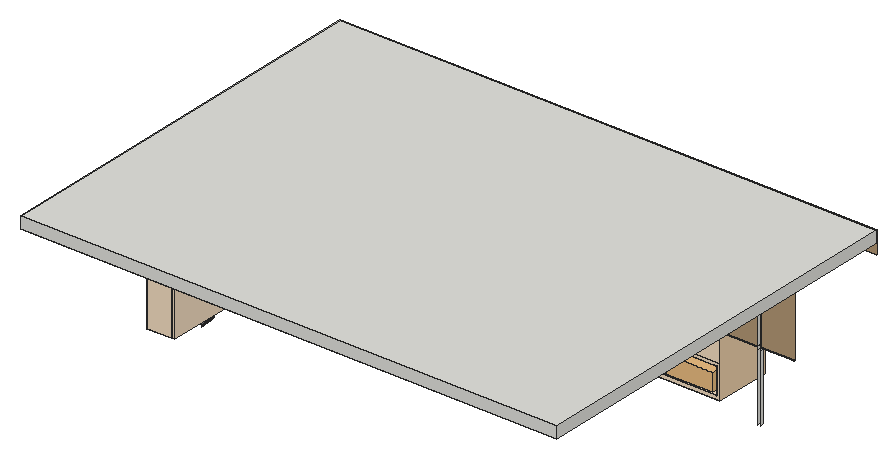
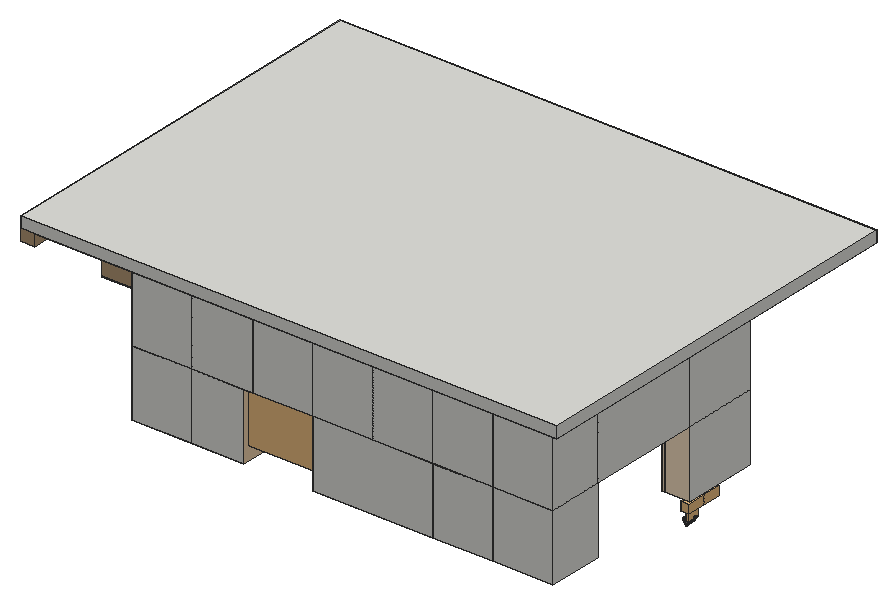
# SketchUp Ruby script. Lengths in inches.
U = 1.inch
M = Sketchup.active_model
def pt(a) = Geom::Point3d.new(a.map { |v| v * U })
def face(e, loops, mat)
  f = e.add_face(loops[0].map { |a| pt(a) })
  loops[1..].each { |l| e.add_face(l.map { |a| pt(a) }).erase! }
  f.material = f.back_material = mat if mat
  f
end
# faces: each face lists its corners as indices into pts; further lists are holes
def faces(e, pts, list, mat = nil) = list.each { |f| face(e, (f[0].is_a?(Array) ? f : [f]).map { |l| l.map { |i| pts[i] } }, mat) }
# xy, xz, yz: faces in a plane at the given z, y or x. An outline is a flat list of corners, or four numbers for a rectangle; further outlines are holes
def ring(l) = l.size == 4 ? [[l[0], l[1]], [l[2], l[1]], [l[2], l[3]], [l[0], l[3]]] : l.each_slice(2).to_a
def flat(e, list, mat, &to3) = list.each { |f| face(e, (f[0].is_a?(Array) ? f : [f]).map { |l| ring(l).map { |u, v| to3.(u, v) } }, mat) }
def xy(e, z, list, mat = nil) = flat(e, list, mat) { |x, y| [x, y, z] }
def xz(e, y, list, mat = nil) = flat(e, list, mat) { |x, z| [x, y, z] }
def yz(e, x, list, mat = nil) = flat(e, list, mat) { |y, z| [x, y, z] }
def lines(e, pts, list) = list.each { |a, b| e.add_line(pt(pts[a]), pt(pts[b])) }
# prism: a flat outline (further loops are holes) pulled along v
def prism(e, loops, v, mat = nil)
  f = face(e, loops, mat); d = Geom::Vector3d.new(v.map { |x| x * U })
  f.pushpull(f.normal.samedirection?(d) ? d.length : -d.length)
end
def box(e, o, s, mat = nil) = prism(e, [[o, [o[0] + s[0], o[1], o[2]], [o[0] + s[0], o[1] + s[1], o[2]], [o[0], o[1] + s[1], o[2]]]], [0, 0, s[2]], mat)
def at(x, y, z, deg = 0) = Geom::Transformation.translation(pt([x, y, z])) * Geom::Transformation.rotation(ORIGIN, Z_AXIS, deg.degrees)
def axes(o, x, y, z) = Geom::Transformation.new([*x, 0, *y, 0, *z, 0, *pt(o).to_a, 1])
def part(name) = M.definitions.add(name)
# library, detail: a bought-in or finely detailed component or shape, given as its bounding box
def library(name, o, s) = part(name).tap { |d| box(d.entities, o, s) }
def detail(e, o, s) = box(e.add_group.entities, o, s)
def put(e, d, t, mat = nil) = e.add_instance(d, t).tap { |i| i.material = mat if mat }
def group(e, t, mat = nil) = e.add_group.tap { |g| g.transformation = t; g.material = mat if mat }.entities
root = M.entities
M.materials.add("Generic").color = [180, 152, 118]
M.materials.add("Generic\#1").color = [237, 208, 170]
M.materials.add("Generic\#2").color = [244, 221, 193]
M.materials.add("[Color M00]").color = [255, 255, 255]
M.materials.add("agda_07_riverina_milk").color = [107, 143, 172]
M.materials.add("go trang").color = [128, 128, 128]
c1 = library("Hanging towel rail",[-9.5,0,-6.64],[9.89,2.15,7.51])
c2 = library("Towel rack",[0,0,0],[10.04,4.25,4.73])
c3 = library("place setting",[6.69,0,0],[21.5,21.5,5.53])
c4 = library("AutoSave_platos+BOWLS",[0,0,0],[6.24,6.24,7.68])
c5 = library("Group\#200",[0,0,0],[25.42,9.79,9.57])
c6 = library("Group\#201",[0,0,0],[3.49,3.49,6.7])
c7 = library("Group\#202",[0,0,0],[3.49,3.49,6.7])
c8 = library("Group\#203",[0,0,0],[3.49,3.49,6.7])
c9 = library("chimney",[0,0,0],[35.95,27.65,32.08])
c10 = library("Group\#513",[0,0,0],[2.91,2.91,4.14])
c11 = part("Component\#71")
xz(c11.entities,0,[[0,0,14.99,43.42]],"agda_07_riverina_milk")
xz(c11.entities,7.5,[[0,46.48,14.99,46.48,14.99,48.87,13.76,50.13,1.23,50.13,0,48.87]],"agda_07_riverina_milk")
xz(c11.entities,14.99,[[0,0,14.99,43.42]],"agda_07_riverina_milk")
yz(c11.entities,0,[[0,0,14.99,43.42]],"agda_07_riverina_milk")
yz(c11.entities,14.99,[[0,0,14.99,43.42]],"agda_07_riverina_milk")
p = [[1.53,7.5,46.07],[0,14.99,43.42],[0,0,43.42],[14.99,0,43.42],[14.99,7.5,46.48],[0,7.5,46.48],
  [13.46,7.5,46.07],[14.99,14.99,43.42]]
faces(c11.entities,p,[[0,1,2],[3,4,5,2],[5,0,2],[6,3,7],[6,4,3],[1,5,4,7],[0,5,1],[4,6,7]],"agda_07_riverina_milk")
c12 = part("Component\#69")
xy(c12.entities,0,[[7.08,5.17,4.88,7.37,4.88,9.5625,12.88,9.5625,12.88,7.37,10.68,5.17]],"agda_07_riverina_milk")
xy(c12.entities,29.07,[[4.98,0.48,12.43,0.48,16.97,5.02,16.97,9.5625,0.44,9.5625,0.44,5.02]],"agda_07_riverina_milk")
xy(c12.entities,30.1,[[4.78,0,12.63,0,17.41,4.78,17.41,9.5625,16.97,9.5625,16.97,5.02,12.43,0.48,4.98,0.48,0.44,5.02,0.44,9.5625,0,9.5625,0,4.78]],"agda_07_riverina_milk")
xz(c12.entities,0.48,[[4.98,29.07,12.43,30.1]],"agda_07_riverina_milk")
yz(c12.entities,0.44,[[5.02,29.07,9.5625,30.1]],"agda_07_riverina_milk")
yz(c12.entities,16.97,[[5.02,29.07,9.5625,30.1]],"agda_07_riverina_milk")
p = [[6.09,2.51,5.81],[2.57,6.04,5.81],[4.88,7.37,0],[7.08,5.17,0],[10.68,5.17,0],[11.88,2.51,5.81],
  [12.88,7.37,0],[15.41,6.04,5.81],[2.57,9.5625,5.81],[4.88,9.5625,0],[12.88,9.5625,0],[15.41,9.5625,5.81],
  [4.78,0,30.1],[0,4.78,30.1],[12.63,0,30.1],[17.41,4.78,30.1],[0,9.5625,30.1],[17.41,9.5625,30.1],
  [0.44,5.02,30.1],[4.98,0.48,30.1],[4.98,0.48,29.07],[0.44,5.02,29.07],[12.43,0.48,30.1],[16.97,5.02,30.1],
  [16.97,5.02,29.07],[12.43,0.48,29.07]]
faces(c12.entities,p,[[0,1,2,3],[4,5,0,3],[6,7,5,4],[1,8,9,2],[7,6,10,11],[0,12,13,1],[5,14,12,0],[7,15,14,5],
  [13,16,8,1],[15,7,11,17],[18,19,20,21],[22,23,24,25]],"agda_07_riverina_milk")
c13 = part("Groep\#9")
put(c13.entities,c12,axes([0,19.13,0],[1,0,0],[0,-1,0],[0,0,1]))
put(c13.entities,c12,at(0,0,0))
c14 = library("Group\#511",[0,0,-0.07],[6.38,6.25,7.32])
c15 = library("Tlon Light 450 Ceiling 152 006",[-8.86,-8.86,-3.78],[17.72,17.72,3.56])
xy(root,63.342,[[11.432,108.349,11.528,114.195]],"go trang")
xy(root,72,[[22.125,74.5,23.625,115]])
xy(root,72,[[73.875,177,139,207],[175.875,177,236.5,207]],"Generic\#1")
xy(root,72,[[9,74.5,22.125,115],[9,177,41.5,207],[41.5,177,73.875,207]],"Generic\#2")
xy(root,74.219,[[11.219,177,39.281,205.9375]],"Generic\#2")
xy(root,88.275,[[177.288,177,204,204.9375],[204,177,234.775,204.9375]],"Generic\#2")
xy(root,89,[[11.219,177,39.281,205.9375]],"Generic\#2")
xy(root,89.7,[[74.175,177,139,177.3]])
xy(root,90,[[73.875,177,74.175,177.3],[74.175,177,139,177.3]])
xy(root,90.5,[[11.219,177,39.281,205.9375]],"Generic\#2")
xy(root,105.781,[[38.6875,177,39.281,205.9375]])
xy(root,105.781,[[11.219,177,38.6875,205.9375]],"Generic\#2")
xy(root,108,[[23.625,74.5,23.625,115,9,115,9,177,38.6875,177,38.6875,74.5],[9,74.5,22.125,115],[22.125,74.5,23.625,115],[38.6875,74.5,41.1875,177],[9,177,41.5,207],
  [41.5,177,73.875,177.3],[74.175,177,139,177.3],[171.5,177,171.8,177.3],[171.8,177,175.875,177.3],[175.875,177,236.5,177.3],
  [41.5,177.3,73.875,207],[106.5,177.3,139,207],[171.5,177.3,175.875,207],[175.875,177.3,204,207],[204,177.3,236.5,207]])
xy(root,108,[[139.3,177,139.3,177.3,139,177.3,139,207,171.5,207,171.5,177]],"Generic\#1")
xy(root,108.3,[[41.5,177,73.875,177.3],[73.875,177,74,177.3],[74.3,177,106.5,177.3],[106.8,177,139,177.3],[171.8,177,204,177.3],
  [204.3,177,236.5,177.3]])
xy(root,109.724,[[239.5625,171,261.8125,171.3],[263.25,171,281.625,171.3]])
xy(root,110.024,[[239.5625,171,261.8125,171.3],[263.25,171,281.625,171.3]])
xy(root,144,[[9,74.5,38.6875,177],[38.6875,74.5,41.1875,177],[9,177,41.5,207],[41.5,177,74,207],[74.3,177,106.5,177,106.5,207,74,207,74,177.3,74.3,177.3],
  [106.8,177,139,177,139,207,106.5,207,106.5,177.3,106.8,177.3],[139.3,177,171.5,177,171.5,207,139,207,139,177.3,139.3,177.3],[171.8,177,204,177,204,207,171.5,207,171.5,177.3,171.8,177.3],[204.3,177,236.5,177,236.5,207,204,207,204,177.3,204.3,177.3]],"Generic\#2")
xy(root,150,[[9,9,9,207,239.5625,207,239.5625,182.261,33.739,182.261,33.739,24.739,264.948,24.739,261.8125,172.303,261.8125,172.375,263.25,172.375,263.25,171,281.625,171,281.625,207,289.6875,207,289.6875,9],[239.5625,171,239.5625,182.261,261.601,182.261,261.8125,172.303,261.8125,171],[263.25,171,263.25,172.375,261.8125,172.375,261.8125,172.303,261.601,182.261,239.5625,182.261,239.5625,207,281.625,207,281.625,171]])
xy(root,150,[[281.625,207,289.6875,216]],"Generic")
xy(root,150,[[0,0,0,216,281.625,216,281.625,207,9,207,9,9,289.6875,9,289.6875,0]],"[Color M00]")
xy(root,153.9375,[[33.739,24.739,33.739,182.261,239.5625,182.261,239.5625,171,261.8125,171,261.8125,172.303,264.948,24.739]])
xy(root,156,[[0,0,289.6875,216]])
xz(root,0,[[0,150,289.6875,156]])
xz(root,24.739,[[33.739,150,228.739,153.9375],[228.739,150,264.948,153.9375]])
xz(root,74.5,[[9,72,22.125,108],[22.125,72,23.625,108],[9,108,38.6875,144],[38.6875,108,41.1875,144]],"Generic\#2")
xz(root,108.349,[[[11.436,60.122,11.532,60.123,11.628,60.129,11.723,60.142,11.817,60.161,11.91,60.186,12.001,60.218,12.09,60.255,12.177,60.298,12.261,60.347,12.341,60.402,12.419,60.461,12.493,60.526,12.5625,60.595,12.628,60.669,12.689,60.747,12.745,60.829,12.796,60.915,12.601,60.516,12.716,60.735,12.822,60.96,12.918,61.189,12.948,61.285,12.972,61.383,12.989,61.483,13.001,61.583,13.007,61.684,13.007,61.785,13.001,61.886,12.989,61.987,12.971,62.086,12.947,62.184,12.917,62.28,12.882,62.374,12.841,62.466,12.794,62.554,12.743,62.64,12.686,62.721,12.625,62.799,12.559,62.873,12.489,62.942,12.415,63.006,12.338,63.066,12.257,63.12,12.173,63.169,12.086,63.211,11.997,63.249,11.906,63.28,11.8125,63.305,11.718,63.324,11.623,63.336,11.528,63.342,11.432,63.342,11.336,63.336,11.241,63.323,11.147,63.304,11.054,63.278,10.963,63.247,10.874,63.21,10.787,63.166,10.703,63.118,10.622,63.063,10.545,63.004,10.471,62.939,10.401,62.87,10.336,62.796,10.275,62.718,10.219,62.636,10.167,62.55,10.121,62.462,10.081,62.37,10.045,62.276,10.016,62.18,9.992,62.081,9.974,61.982,9.963,61.882,9.963,61.881,9.961,61.858,9.957,61.781,9.957,61.68,9.963,61.579,9.975,61.478,9.993,61.379,10.017,61.281,10.047,61.185,10.082,61.091,10.123,60.999,10.17,60.911,10.221,60.825,10.278,60.743,10.339,60.666,10.404,60.592,10.474,60.523,10.548,60.458,10.626,60.399,10.707,60.345,10.791,60.296,10.878,60.253,10.967,60.216,11.058,60.185,11.151,60.16,11.245,60.141,11.34,60.129],[11.482,61.122,11.446,61.124,11.409,61.127,11.374,61.133,11.338,61.142,11.303,61.152,11.269,61.165,11.236,61.18,11.203,61.198,11.172,61.217,11.142,61.239,11.114,61.262,11.086,61.288,11.061,61.315,11.037,61.344,11.014,61.374,10.994,61.406,10.975,61.439,10.959,61.473,10.945,61.508,10.932,61.544,10.922,61.581,10.914,61.618,10.909,61.656,10.905,61.694,10.904,61.732,10.905,61.771,10.909,61.809,10.914,61.847,10.922,61.884,10.932,61.921,10.945,61.957,10.959,61.992,10.975,62.026,10.994,62.059,11.014,62.091,11.037,62.121,11.061,62.15,11.086,62.177,11.114,62.202,11.142,62.226,11.172,62.247,11.203,62.267,11.236,62.284,11.269,62.3,11.303,62.3125,11.338,62.323,11.374,62.332,11.409,62.338,11.446,62.341,11.482,62.342,11.518,62.341,11.554,62.338,11.59,62.332,11.626,62.323,11.661,62.3125,11.695,62.3,11.728,62.284,11.76,62.267,11.792,62.247,11.822,62.226,11.85,62.202,11.878,62.177,11.903,62.15,11.927,62.121,11.95,62.091,11.97,62.059,11.988,62.026,12.005,61.992,12.019,61.957,12.032,61.921,12.042,61.884,12.05,61.847,12.055,61.809,12.059,61.771,12.06,61.732,12.059,61.694,12.055,61.656,12.05,61.618,12.042,61.581,12.032,61.544,12.019,61.508,12.005,61.473,11.988,61.439,11.97,61.406,11.95,61.374,11.927,61.344,11.903,61.315,11.878,61.288,11.85,61.262,11.822,61.239,11.792,61.217,11.76,61.198,11.728,61.18,11.695,61.165,11.661,61.152,11.626,61.142,11.59,61.133,11.554,61.127,11.518,61.124]],[12.601,60.516,12.716,60.735,12.822,60.96,12.918,61.189,12.883,61.095,12.843,61.003,12.796,60.915]],"go trang")
xz(root,114.195,[[[11.436,60.122,11.34,60.129,11.245,60.141,11.151,60.16,11.058,60.185,10.967,60.216,10.878,60.253,10.791,60.296,10.707,60.345,10.626,60.399,10.548,60.458,10.474,60.523,10.404,60.592,10.339,60.666,10.278,60.743,10.221,60.825,10.17,60.911,10.123,60.999,10.082,61.091,10.047,61.185,10.017,61.281,9.993,61.379,9.975,61.478,9.963,61.579,9.957,61.68,9.957,61.781,9.961,61.858,9.963,61.881,9.963,61.882,9.974,61.982,9.992,62.081,10.016,62.18,10.045,62.276,10.081,62.37,10.121,62.462,10.167,62.55,10.219,62.636,10.275,62.718,10.336,62.796,10.401,62.87,10.471,62.939,10.545,63.004,10.622,63.063,10.703,63.118,10.787,63.166,10.874,63.21,10.963,63.247,11.054,63.278,11.147,63.304,11.241,63.323,11.336,63.336,11.432,63.342,11.528,63.342,11.623,63.336,11.718,63.324,11.8125,63.305,11.906,63.28,11.997,63.249,12.086,63.211,12.173,63.169,12.257,63.12,12.338,63.066,12.415,63.006,12.489,62.942,12.559,62.873,12.625,62.799,12.686,62.721,12.743,62.64,12.794,62.554,12.841,62.466,12.882,62.374,12.917,62.28,12.947,62.184,12.971,62.086,12.989,61.987,13.001,61.886,13.007,61.785,13.007,61.684,13.001,61.583,12.989,61.483,12.972,61.383,12.948,61.285,12.918,61.189,12.883,61.095,12.843,61.003,12.796,60.915,12.745,60.829,12.689,60.747,12.628,60.669,12.5625,60.595,12.493,60.526,12.419,60.461,12.341,60.402,12.261,60.347,12.177,60.298,12.09,60.255,12.001,60.218,11.91,60.186,11.817,60.161,11.723,60.142,11.628,60.129,11.532,60.123],[11.482,61.122,11.518,61.124,11.554,61.127,11.59,61.133,11.626,61.142,11.661,61.152,11.695,61.165,11.728,61.18,11.76,61.198,11.792,61.217,11.822,61.239,11.85,61.262,11.878,61.288,11.903,61.315,11.927,61.344,11.95,61.374,11.97,61.406,11.988,61.439,12.005,61.473,12.019,61.508,12.032,61.544,12.042,61.581,12.05,61.618,12.055,61.656,12.059,61.694,12.06,61.732,12.059,61.771,12.055,61.809,12.05,61.847,12.042,61.884,12.032,61.921,12.019,61.957,12.005,61.992,11.988,62.026,11.97,62.059,11.95,62.091,11.927,62.121,11.903,62.15,11.878,62.177,11.85,62.202,11.822,62.226,11.792,62.247,11.76,62.267,11.728,62.284,11.695,62.3,11.661,62.3125,11.626,62.323,11.59,62.332,11.554,62.338,11.518,62.341,11.482,62.342,11.446,62.341,11.409,62.338,11.374,62.332,11.338,62.323,11.303,62.3125,11.269,62.3,11.236,62.284,11.203,62.267,11.172,62.247,11.142,62.226,11.114,62.202,11.086,62.177,11.061,62.15,11.037,62.121,11.014,62.091,10.994,62.059,10.975,62.026,10.959,61.992,10.945,61.957,10.932,61.921,10.922,61.884,10.914,61.847,10.909,61.809,10.905,61.771,10.904,61.732,10.905,61.694,10.909,61.656,10.914,61.618,10.922,61.581,10.932,61.544,10.945,61.508,10.959,61.473,10.975,61.439,10.994,61.406,11.014,61.374,11.037,61.344,11.061,61.315,11.086,61.288,11.114,61.262,11.142,61.239,11.172,61.217,11.203,61.198,11.236,61.18,11.269,61.165,11.303,61.152,11.338,61.142,11.374,61.133,11.409,61.127,11.446,61.124]],[12.416,60.337,12.419,60.461,12.493,60.526,12.5625,60.595,12.628,60.669,12.523,60.502]],"go trang")
xz(root,115,[[9,72,22.125,108],[22.125,72,23.625,108]],"Generic\#2")
xz(root,171,[[239.5625,150,261.8125,153.9375]])
xz(root,171,[[239.5625,110.024,261.8125,150],[263.25,110.024,281.625,150]],"Generic")
xz(root,171.3,[[239.5625,109.724,261.8125,110.024],[263.25,109.724,281.625,110.024]])
xz(root,177,[[73.875,72,74.175,90],[9,108,38.6875,144],[38.6875,108,41.1875,144],[41.1875,108,41.5,144]])
xz(root,177,[[[9,72,41.5,108],[11.219,90.5,39.281,105.781],[11.219,74.219,39.281,89]],[41.5,72,73.875,108],[74.175,72,139,89.7],[[175.875,72,236.5,90],[177.288,73.725,234.775,88.275]],[74.175,90,139,108],
  [175.875,90,236.5,108],[139.3,108,171.5,144],[41.5,108.3,74,144],[74.3,108.3,106.5,144],[106.8,108.3,139,144],
  [171.8,108.3,204,144],[204.3,108.3,236.5,144]],"Generic\#2")
xz(root,177.3,[[74.175,89.7,139,90],[73.875,90,74.175,90,74.175,108,139.3,108,139.3,144,139,144,139,108.3,106.8,108.3,106.8,144,106.5,144,106.5,108.3,74.3,108.3,74.3,144,74,144,74,108.3,41.5,108.3,41.5,108,73.875,108],[171.5,108,236.5,108,236.5,108.3,204.3,108.3,204.3,144,204,144,204,108.3,171.8,108.3,171.8,144,171.5,144]])
xz(root,182.261,[[33.739,150,235.163,153.9375],[235.163,150,239.5625,153.9375]])
xz(root,204.9375,[[177.288,73.725,234.775,88.275]],"Generic\#2")
xz(root,205.9375,[[11.219,74.219,39.281,89],[11.219,90.5,39.281,105.781]],"Generic\#2")
xz(root,207,[[9,72,41.5,108],[41.5,72,73.875,108],[73.875,72,139,108],[175.875,72,204,108],[204,72,236.5,108],
  [9,108,41.5,144],[41.5,108,74,144],[74,108,106.5,144],[106.5,108,139,144],[139,108,171.5,144],
  [171.5,108,204,144],[204,108,236.5,144]])
xz(root,207,[[9,144,236.5,150]],"[Color M00]")
xz(root,216,[[0,150,289.6875,156]])
xz(root,216,[[281.625,144,289.6875,150]],"Generic")
yz(root,0,[[0,150,216,156]])
yz(root,9,[[74.5,72,115,108],[177,72,207,108],[74.5,108,115,144],[115,108,177,144],[177,108,207,144]])
yz(root,9.957,[[108.349,61.68,114.195,61.781]],"go trang")
yz(root,9.963,[[108.349,61.881,114.195,61.882]],"go trang")
yz(root,11.219,[[177,74.219,205.9375,89],[177,90.5,205.9375,105.781]],"Generic\#2")
yz(root,13.007,[[108.349,61.684,114.195,61.785]],"go trang")
yz(root,22.125,[[74.5,72,115,108]])
yz(root,23.625,[[74.5,72,115,108]],"Generic\#2")
yz(root,33.739,[[24.739,150,182.261,153.9375]])
yz(root,38.6875,[[74.5,108,177,144]])
yz(root,39.281,[[177,89,205.9375,90.5]])
yz(root,39.281,[[177,74.219,205.9375,89],[177,90.5,205.9375,105.781]],"Generic\#2")
yz(root,41.1875,[[74.5,108,177,144]],"Generic\#2")
yz(root,41.5,[[177,72,207,108],[177,108,177.3,108.3],[177.3,108,177.3,108.3,177,108.3,177,144,207,144,207,108]])
yz(root,73.875,[[177,72,207,72,207,108,177.3,108,177.3,90,177,90],[177,90,177.3,108]])
yz(root,74,[[177,108.3,177.3,144]])
yz(root,74.175,[[177,89.7,177.3,90],[177,90,177.3,108]])
yz(root,74.3,[[177,108.3,177.3,144]])
yz(root,106.5,[[177,108.3,177.3,144]])
yz(root,106.8,[[177,108.3,177.3,144]])
yz(root,139,[[177,108.3,177.3,144]])
yz(root,139,[[177,72,207,72,207,108,177,108,177,90,177.3,90,177.3,89.7,177,89.7]],"Generic\#2")
yz(root,139.3,[[177,108,177.3,144]])
yz(root,171.5,[[177,108,177.3,144],[177.3,108,207,144]])
yz(root,171.8,[[177,108.3,177.3,144]])
yz(root,175.875,[[177,72,207,108]],"Generic\#1")
yz(root,177.288,[[177,73.725,204.9375,88.275]],"Generic\#2")
yz(root,204,[[177,108.3,177.3,144]])
yz(root,204.3,[[177,108.3,177.3,144]])
yz(root,234.775,[[177,73.725,204.9375,88.275]],"Generic\#2")
yz(root,236.5,[[177,72,207,108],[177.3,108,207,108,207,144,177,144,177,108.3,177.3,108.3]],"Generic\#1")
yz(root,239.5625,[[171,150,182.261,153.9375]])
yz(root,261.8125,[[171,72,172.375,108],[171,108,172.375,109.724],[171.3,109.724,172.375,110.024],[171,110.024,172.375,150],[171,150,172.303,153.9375]])
yz(root,263.25,[[171,72,172.375,108],[171,108,172.375,109.724],[171.3,109.724,172.375,110.024],[171,110.024,172.375,150]])
yz(root,281.625,[[207,144,216,150]],"Generic")
yz(root,289.6875,[[0,150,216,156]])
p = [[11.176,114.195,58.811],[11.365,108.349,58.972],[11.176,108.349,58.811],[11.3125,114.195,58.953],[11.447,114.195,59.097],[11.547,108.349,59.14],
  [11.722,108.349,59.317],[11.578,114.195,59.244],[11.889,108.349,59.5],[11.706,114.195,59.393],[12.049,108.349,59.691],[12.2,108.349,59.888],
  [11.832,114.195,59.545],[11.955,114.195,59.699],[12.074,114.195,59.855],[12.342,108.349,60.091],[12.191,114.195,60.014],[12.305,114.195,60.174],
  [11.245,114.195,60.141],[11.34,114.195,60.129],[11.34,108.349,60.129],[11.245,108.349,60.141],[11.151,114.195,60.16],[11.151,108.349,60.16],
  [11.436,114.195,60.122],[11.436,108.349,60.122],[11.532,114.195,60.123],[11.532,108.349,60.123],[11.628,114.195,60.129],[11.628,108.349,60.129],
  [11.723,114.195,60.142],[11.723,108.349,60.142],[11.817,114.195,60.161],[11.817,108.349,60.161],[12.476,108.349,60.301],[10.878,114.195,60.253],
  [10.967,114.195,60.216],[10.967,108.349,60.216],[10.878,108.349,60.253],[11.058,114.195,60.185],[11.058,108.349,60.185],[11.91,114.195,60.186],
  [11.91,108.349,60.186],[12.001,114.195,60.218],[12.001,108.349,60.218],[12.09,114.195,60.255],[12.09,108.349,60.255],[12.416,114.195,60.337],
  [10.626,114.195,60.399],[10.707,114.195,60.345],[10.707,108.349,60.345],[10.626,108.349,60.399],[10.791,114.195,60.296],[10.791,108.349,60.296],
  [12.177,114.195,60.298],[12.177,108.349,60.298],[12.261,114.195,60.347],[12.261,108.349,60.347],[12.341,114.195,60.402],[12.341,108.349,60.402],
  [12.538,108.349,60.408],[12.523,114.195,60.502],[10.548,114.195,60.458],[10.548,108.349,60.458],[12.419,114.195,60.461],[12.419,108.349,60.461],
  [12.601,108.349,60.516],[10.404,114.195,60.592],[10.474,114.195,60.523],[10.474,108.349,60.523],[10.404,108.349,60.592],[12.493,114.195,60.526],
  [12.493,108.349,60.526],[12.628,114.195,60.669],[12.5625,114.195,60.595],[12.5625,108.349,60.595],[12.716,108.349,60.735],[10.339,114.195,60.666],
  [10.339,108.349,60.666],[12.628,108.349,60.669],[10.221,114.195,60.825],[10.278,114.195,60.743],[10.278,108.349,60.743],[10.221,108.349,60.825],
  [12.689,114.195,60.747],[12.689,108.349,60.747],[12.745,114.195,60.829],[12.745,108.349,60.829],[10.17,114.195,60.911],[10.17,108.349,60.911],
  [12.796,114.195,60.915],[12.796,108.349,60.915],[10.123,114.195,60.999],[10.123,108.349,60.999],[12.843,114.195,61.003],[12.843,108.349,61.003],
  [10.082,114.195,61.091],[10.082,108.349,61.091],[12.883,114.195,61.095],[12.883,108.349,61.095],[10.047,114.195,61.185],[10.047,108.349,61.185],
  [11.374,114.195,61.133],[11.338,114.195,61.142],[11.338,108.349,61.142],[11.374,108.349,61.133],[11.303,114.195,61.152],[11.303,108.349,61.152],
  [11.482,114.195,61.122],[11.446,114.195,61.124],[11.446,108.349,61.124],[11.482,108.349,61.122],[11.409,114.195,61.127],[11.409,108.349,61.127],
  [11.518,114.195,61.124],[11.518,108.349,61.124],[11.554,114.195,61.127],[11.554,108.349,61.127],[11.59,114.195,61.133],[11.59,108.349,61.133],
  [11.626,114.195,61.142],[11.626,108.349,61.142],[11.661,114.195,61.152],[11.661,108.349,61.152],[12.918,114.195,61.189],[12.918,108.349,61.189],
  [10.017,114.195,61.281],[10.017,108.349,61.281],[11.172,114.195,61.217],[11.142,114.195,61.239],[11.142,108.349,61.239],[11.172,108.349,61.217],
  [11.114,114.195,61.262],[11.114,108.349,61.262],[11.269,114.195,61.165],[11.236,114.195,61.18],[11.236,108.349,61.18],[11.269,108.349,61.165],
  [11.203,114.195,61.198],[11.203,108.349,61.198],[11.695,114.195,61.165],[11.695,108.349,61.165],[11.728,114.195,61.18],[11.728,108.349,61.18],
  [11.76,114.195,61.198],[11.76,108.349,61.198],[11.792,114.195,61.217],[11.792,108.349,61.217],[11.822,114.195,61.239],[11.822,108.349,61.239],
  [11.85,114.195,61.262],[11.85,108.349,61.262],[12.948,114.195,61.285],[12.948,108.349,61.285],[9.993,114.195,61.379],[9.993,108.349,61.379],
  [11.061,114.195,61.315],[11.037,114.195,61.344],[11.037,108.349,61.344],[11.061,108.349,61.315],[11.014,114.195,61.374],[11.014,108.349,61.374],
  [11.086,114.195,61.288],[11.086,108.349,61.288],[11.878,114.195,61.288],[11.878,108.349,61.288],[11.903,114.195,61.315],[11.903,108.349,61.315],
  [11.927,114.195,61.344],[11.927,108.349,61.344],[11.95,114.195,61.374],[11.95,108.349,61.374],[12.972,114.195,61.383],[12.972,108.349,61.383],
  [9.975,114.195,61.478],[9.975,108.349,61.478],[10.994,114.195,61.406],[10.994,108.349,61.406],[10.975,114.195,61.439],[10.975,108.349,61.439],
  [10.959,114.195,61.473],[10.959,108.349,61.473],[11.97,114.195,61.406],[11.97,108.349,61.406],[11.988,114.195,61.439],[11.988,108.349,61.439],
  [12.005,114.195,61.473],[12.005,108.349,61.473],[12.989,114.195,61.483],[12.989,108.349,61.483],[9.963,114.195,61.579],[9.963,108.349,61.579],
  [10.945,114.195,61.508],[10.945,108.349,61.508],[10.932,114.195,61.544],[10.932,108.349,61.544],[10.922,114.195,61.581],[10.922,108.349,61.581],
  [12.019,114.195,61.508],[12.019,108.349,61.508],[12.032,114.195,61.544],[12.032,108.349,61.544],[12.042,114.195,61.581],[12.042,108.349,61.581],
  [13.001,114.195,61.583],[13.001,108.349,61.583],[9.957,114.195,61.68],[9.957,108.349,61.68],[10.914,114.195,61.618],[10.914,108.349,61.618],
  [10.909,114.195,61.656],[10.909,108.349,61.656],[12.05,114.195,61.618],[12.05,108.349,61.618],[12.055,114.195,61.656],[12.055,108.349,61.656],
  [13.007,114.195,61.684],[13.007,108.349,61.684],[10.905,114.195,61.694],[10.905,108.349,61.694],[10.904,114.195,61.732],[10.904,108.349,61.732],
  [10.905,114.195,61.771],[10.905,108.349,61.771],[12.059,114.195,61.694],[12.059,108.349,61.694],[12.06,114.195,61.732],[12.06,108.349,61.732],
  [12.059,114.195,61.771],[12.059,108.349,61.771],[9.957,108.349,61.781],[9.961,108.349,61.858],[9.961,114.195,61.858],[9.957,114.195,61.781],
  [10.909,114.195,61.809],[10.909,108.349,61.809],[10.914,114.195,61.847],[10.914,108.349,61.847],[10.922,114.195,61.884],[10.922,108.349,61.884],
  [12.05,114.195,61.847],[12.055,114.195,61.809],[12.055,108.349,61.809],[12.05,108.349,61.847],[12.042,114.195,61.884],[12.042,108.349,61.884],
  [13.007,114.195,61.785],[13.001,114.195,61.886],[13.001,108.349,61.886],[13.007,108.349,61.785],[9.963,114.195,61.881],[9.963,108.349,61.881],
  [9.974,114.195,61.982],[9.963,114.195,61.882],[9.963,114.175,61.882],[9.963,108.349,61.882],[9.974,108.349,61.982],[10.932,114.195,61.921],
  [10.932,108.349,61.921],[10.945,114.195,61.957],[10.945,108.349,61.957],[12.032,114.195,61.921],[12.032,108.349,61.921],[12.019,114.195,61.957],
  [12.019,108.349,61.957],[12.989,114.195,61.987],[12.989,108.349,61.987],[9.992,114.195,62.081],[9.992,108.349,62.081],[10.959,114.195,61.992],
  [10.959,108.349,61.992],[10.975,114.195,62.026],[10.975,108.349,62.026],[10.994,114.195,62.059],[10.994,108.349,62.059],[12.005,114.195,61.992],
  [12.005,108.349,61.992],[11.988,114.195,62.026],[11.988,108.349,62.026],[11.97,114.195,62.059],[11.97,108.349,62.059],[12.971,114.195,62.086],
  [12.971,108.349,62.086],[10.016,114.195,62.18],[10.016,108.349,62.18],[11.014,114.195,62.091],[11.014,108.349,62.091],[11.037,114.195,62.121],
  [11.037,108.349,62.121],[11.061,114.195,62.15],[11.061,108.349,62.15],[11.086,114.195,62.177],[11.086,108.349,62.177],[11.95,114.195,62.091],
  [11.95,108.349,62.091],[11.927,114.195,62.121],[11.927,108.349,62.121],[11.903,114.195,62.15],[11.903,108.349,62.15],[11.878,114.195,62.177],
  [11.878,108.349,62.177],[12.947,114.195,62.184],[12.947,108.349,62.184],[10.045,114.195,62.276],[10.045,108.349,62.276],[11.114,114.195,62.202],
  [11.114,108.349,62.202],[11.142,114.195,62.226],[11.142,108.349,62.226],[11.172,114.195,62.247],[11.172,108.349,62.247],[11.203,114.195,62.267],
  [11.203,108.349,62.267],[11.822,114.195,62.226],[11.85,114.195,62.202],[11.85,108.349,62.202],[11.822,108.349,62.226],[11.792,114.195,62.247],
  [11.792,108.349,62.247],[11.76,114.195,62.267],[11.76,108.349,62.267],[12.917,114.195,62.28],[12.917,108.349,62.28],[10.081,114.195,62.37],
  [10.081,108.349,62.37],[11.236,114.195,62.284],[11.236,108.349,62.284],[11.269,114.195,62.3],[11.269,108.349,62.3],[11.303,114.195,62.3125],
  [11.303,108.349,62.3125],[11.338,114.195,62.323],[11.338,108.349,62.323],[11.374,114.195,62.332],[11.374,108.349,62.332],[11.409,114.195,62.338],
  [11.409,108.349,62.338],[11.446,114.195,62.341],[11.446,108.349,62.341],[11.482,114.195,62.342],[11.482,108.349,62.342],[11.518,114.195,62.341],
  [11.554,114.195,62.338],[11.554,108.349,62.338],[11.518,108.349,62.341],[11.626,114.195,62.323],[11.661,114.195,62.3125],[11.661,108.349,62.3125],
  [11.626,108.349,62.323],[11.59,114.195,62.332],[11.59,108.349,62.332],[11.728,114.195,62.284],[11.728,108.349,62.284],[11.695,114.195,62.3],
  [11.695,108.349,62.3],[12.882,114.195,62.374],[12.882,108.349,62.374],[10.121,114.195,62.462],[10.121,108.349,62.462],[12.841,114.195,62.466],
  [12.841,108.349,62.466],[10.167,114.195,62.55],[10.167,108.349,62.55],[12.794,114.195,62.554],[12.794,108.349,62.554],[10.219,114.195,62.636],
  [10.219,108.349,62.636],[10.275,114.195,62.718],[10.275,108.349,62.718],[12.743,114.195,62.64],[12.743,108.349,62.64],[12.686,114.195,62.721],
  [12.686,108.349,62.721],[10.336,114.195,62.796],[10.336,108.349,62.796],[12.625,114.195,62.799],[12.625,108.349,62.799],[10.401,114.195,62.87],
  [10.401,108.349,62.87],[12.559,114.195,62.873],[12.559,108.349,62.873],[10.471,114.195,62.939],[10.471,108.349,62.939],[10.545,114.195,63.004],
  [10.545,108.349,63.004],[12.489,114.195,62.942],[12.415,114.195,63.006],[12.415,108.349,63.006],[12.489,108.349,62.942],[10.622,114.195,63.063],
  [10.622,108.349,63.063],[12.338,114.195,63.066],[12.338,108.349,63.066],[10.703,114.195,63.118],[10.703,108.349,63.118],[10.787,114.195,63.166],
  [10.787,108.349,63.166],[12.257,114.195,63.12],[12.173,114.195,63.169],[12.173,108.349,63.169],[12.257,108.349,63.12],[10.874,114.195,63.21],
  [10.874,108.349,63.21],[10.963,114.195,63.247],[10.963,108.349,63.247],[11.054,114.195,63.278],[11.054,108.349,63.278],[11.997,114.195,63.249],
  [11.906,114.195,63.28],[11.906,108.349,63.28],[11.997,108.349,63.249],[12.086,114.195,63.211],[12.086,108.349,63.211],[11.147,114.195,63.304],
  [11.147,108.349,63.304],[11.241,114.195,63.323],[11.241,108.349,63.323],[11.336,114.195,63.336],[11.336,108.349,63.336],[11.432,114.195,63.342],
  [11.432,108.349,63.342],[11.623,114.195,63.336],[11.528,114.195,63.342],[11.528,108.349,63.342],[11.623,108.349,63.336],[11.718,114.195,63.324],
  [11.718,108.349,63.324],[11.8125,114.195,63.305],[11.8125,108.349,63.305],[261.8125,172.303,150],[264.948,24.739,150],[264.948,24.739,153.9375],
  [261.8125,172.303,153.9375],[10.324,79,71.206],[10.322,79,71.222]]
faces(root,p,[[0,1,2],[1,0,3],[4,5,3],[3,5,1],[4,6,5],[7,6,4],[7,8,6],[9,8,7],
  [9,10,11],[10,9,8],[11,12,9],[11,13,12],[11,14,13],[15,14,11],[16,15,14],[15,16,17],
  [18,19,20,21],[22,18,21,23],[19,24,25,20],[24,26,27,25],[26,28,29,27],[28,30,31,29],[30,32,33,31],[17,34,15],
  [35,36,37,38],[36,39,40,37],[39,22,23,40],[32,41,42,33],[41,43,44,42],[43,45,46,44],[47,34,17],[48,49,50,51],
  [49,52,53,50],[52,35,38,53],[45,54,55,46],[54,56,57,55],[56,58,59,57],[47,60,34],[61,60,47],[62,48,51,63],
  [58,64,65,59],[61,66,60],[67,68,69,70],[68,62,63,69],[64,71,72,65],[73,66,61],[71,74,75,72],[73,76,66],
  [77,67,70,78],[73,79,75,74],[80,81,82,83],[81,77,78,82],[73,84,85,79],[76,73,84],[84,86,87,85],[88,80,83,89],
  [86,90,91,87],[92,88,89,93],[90,94,95,91],[96,92,93,97],[94,98,99,95],[100,96,97,101],[102,103,104,105],[103,106,107,104],
  [108,109,110,111],[109,112,113,110],[112,102,105,113],[114,108,111,115],[116,114,115,117],[118,116,117,119],[120,118,119,121],[122,120,121,123],
  [98,124,125,99],[126,100,101,127],[128,129,130,131],[129,132,133,130],[134,135,136,137],[135,138,139,136],[138,128,131,139],[106,134,137,107],
  [140,122,123,141],[142,140,141,143],[144,142,143,145],[146,144,145,147],[148,146,147,149],[150,148,149,151],[124,152,153,125],[154,126,127,155],
  [156,157,158,159],[157,160,161,158],[132,162,163,133],[162,156,159,163],[164,150,151,165],[166,164,165,167],[168,166,167,169],[170,168,169,171],
  [152,172,173,153],[174,154,155,175],[160,176,177,161],[176,178,179,177],[178,180,181,179],[182,170,171,183],[184,182,183,185],[186,184,185,187],
  [172,188,189,173],[190,174,175,191],[180,192,193,181],[192,194,195,193],[194,196,197,195],[198,186,187,199],[200,198,199,201],[202,200,201,203],
  [188,204,205,189],[206,190,191,207],[196,208,209,197],[208,210,211,209],[212,202,203,213],[214,212,213,215],[204,216,217,205],[210,218,219,211],
  [218,220,221,219],[220,222,223,221],[224,214,215,225],[226,224,225,227],[228,226,227,229],[230,231,232,233],[222,234,235,223],[234,236,237,235],
  [236,238,239,237],[240,241,242,243],[244,240,243,245],[241,228,229,242],[246,247,248,249],[250,232,231,251],[252,253,254,255,256],[238,257,258,239],
  [257,259,260,258],[261,244,245,262],[263,261,262,264],[247,265,266,248],[267,252,256,268],[259,269,270,260],[269,271,272,270],[271,273,274,272],
  [275,263,264,276],[277,275,276,278],[279,277,278,280],[265,281,282,266],[283,267,268,284],[273,285,286,274],[285,287,288,286],[287,289,290,288],
  [289,291,292,290],[293,279,280,294],[295,293,294,296],[297,295,296,298],[299,297,298,300],[281,301,302,282],[303,283,284,304],[291,305,306,292],
  [305,307,308,306],[307,309,310,308],[309,311,312,310],[313,314,315,316],[317,313,316,318],[319,317,318,320],[314,299,300,315],[301,321,322,302],
  [323,303,304,324],[311,325,326,312],[325,327,328,326],[327,329,330,328],[329,331,332,330],[331,333,334,332],[333,335,336,334],[335,337,338,336],
  [337,339,340,338],[341,342,343,344],[339,341,344,340],[345,346,347,348],[349,345,348,350],[342,349,350,343],[351,319,320,352],[353,351,352,354],
  [346,353,354,347],[321,355,356,322],[357,323,324,358],[355,359,360,356],[361,357,358,362],[359,363,364,360],[365,361,362,366],[367,365,366,368],
  [363,369,370,364],[369,371,372,370],[373,367,368,374],[371,375,376,372],[377,373,374,378],[375,379,380,376],[381,377,378,382],[383,381,382,384],
  [385,386,387,388],[379,385,388,380],[389,383,384,390],[386,391,392,387],[393,389,390,394],[395,393,394,396],[397,398,399,400],[391,397,400,392],
  [401,395,396,402],[403,401,402,404],[405,403,404,406],[407,408,409,410],[411,407,410,412],[398,411,412,399],[413,405,406,414],[415,413,414,416],
  [417,415,416,418],[419,417,418,420],[421,422,423,424],[425,421,424,426],[427,425,426,428],[408,427,428,409]],"go trang")
faces(root,p,[[429,430,431,432]])
lines(root,p,[[433,434],[98,153],[90,99],[84,91]])
put(root,c1,axes([9.9,108.38,65.73],[0,-0.64,0],[0.64,0,0],[0,0,0.64]),"go trang")
put(root,c2,axes([13.26,105.3125,65.98],[0,-1,0],[-1,0,0],[0,0,1]),"go trang")
put(root,c2,at(13.26,105.3125,65.98,90),"go trang")
put(root,c3,axes([191.67,197.3,73.73],[0,-0.66792,0],[0.66792,0,0],[0,0,0.82154]))
g1 = group(root,at(177.29,177,73.73),"Generic\#2")
xy(g1,0,[[0,0,57.49,27.9375]])
put(root,c4,axes([182.06,180.17,73.73],[1.32,0,0],[0,1.32,0],[0,0,1.32]),"Generic\#2")
put(root,c5,at(206.04,178.36,73.73))
put(root,c6,axes([12.68,187.2,74.22],[0,-1.9551,0],[1.9551,0,0],[0,0,1.9551]))
put(root,c7,axes([21.06,187.04,74.22],[0,-1.9404,0],[1.9404,0,0],[0,0,1.9404]))
put(root,c8,axes([29.48,187.25,74.22],[0,-1.9992,0],[1.9992,0,0],[0,0,1.9992]))
put(root,c3,axes([191.67,197.3,76.35],[0,-0.66792,0],[0.66792,0,0],[0,0,0.82154]))
put(root,c3,axes([191.67,197.3,78.98],[0,-0.66792,0],[0.66792,0,0],[0,0,0.82154]))
put(root,c9,at(140.33,177,80))
put(root,c10,axes([28.18,180.44,90.5],[1.44889,-0.38823,0],[0.38823,1.44889,0],[0,0,1.5]))
put(root,c10,axes([33.06,180.44,90.5],[1.44889,-0.38823,0],[0.38823,1.44889,0],[0,0,1.5]))
g2 = group(root,at(22.59,185.7,90.5))
put(g2,c11,axes([-5.74,-1.45,0],[-0.2925,0,0],[0,-0.2925,0],[0,0,0.2925]))
put(g2,c13,axes([-0.9,0,0.4],[-0.22034,0,0],[0,-0.22034,0],[0,0,0.22034]))
put(root,c14,at(22.39,179.98,90.57,3.7))
put(root,c15,axes([278.5625,68.67,150.35],[0.39,0,0],[0,0.39,0],[0,0,0.39]))
put(root,c15,axes([278.5625,139.92,150.35],[0.39,0,0],[0,0.39,0],[0,0,0.39]))
put(root,c15,axes([22.33,57.51,150.48],[0.39,0,0],[0,0.39,0],[0,0,0.39]))
put(root,c15,axes([22.33,183.26,150.48],[0.39,0,0],[0,0.39,0],[0,0,0.39]))
put(root,c15,axes([22.33,117.64,150.48],[0.39,0,0],[0,0.39,0],[0,0,0.39]))
put(root,c15,axes([200.17,192.59,150.66],[0.39,0,0],[0,0.39,0],[0,0,0.39]))
put(root,c15,axes([79.36,192.96,150.66],[0.39,0,0],[0,0.39,0],[0,0,0.39]))
put(root,c15,axes([142.17,192.96,150.66],[0.39,0,0],[0,0.39,0],[0,0,0.39]))
put(root,c15,axes([45.67,17.96,150.78],[0.39,0,0],[0,0.39,0],[0,0,0.39]))
put(root,c15,axes([176.85,17.96,150.78],[0.39,0,0],[0,0.39,0],[0,0,0.39]))
put(root,c15,axes([268.42,17.96,150.78],[0.39,0,0],[0,0.39,0],[0,0,0.39]))
